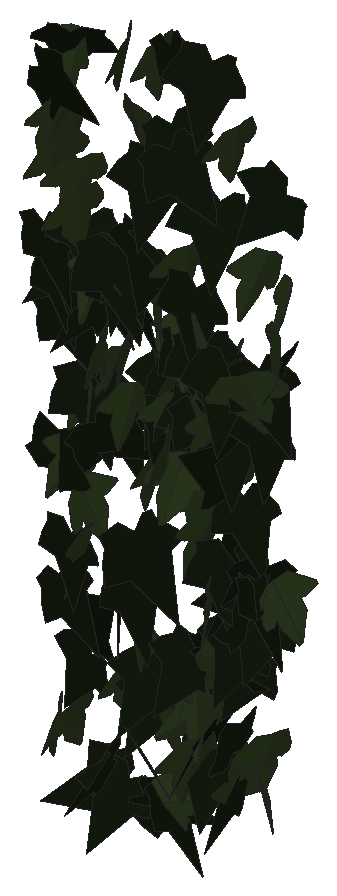
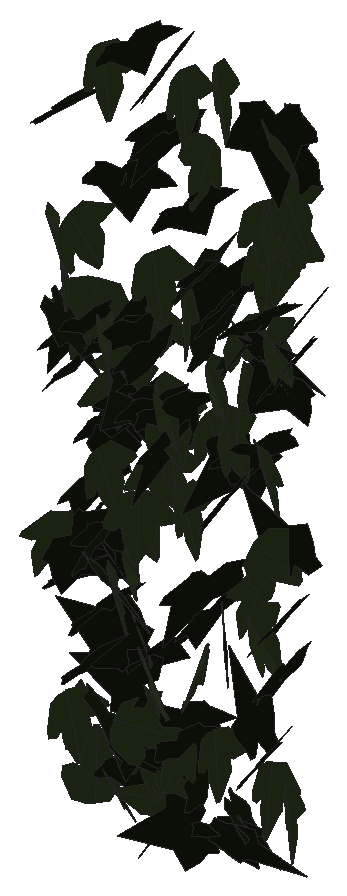
# SketchUp Ruby script. Lengths in inches.
U = 1.inch
M = Sketchup.active_model
def pt(a) = Geom::Point3d.new(a.map { |v| v * U })
def face(e, loops, mat)
  f = e.add_face(loops[0].map { |a| pt(a) })
  loops[1..].each { |l| e.add_face(l.map { |a| pt(a) }).erase! }
  f.material = f.back_material = mat if mat
  f
end
# faces: each face lists its corners as indices into pts; further lists are holes
def faces(e, pts, list, mat = nil) = list.each { |f| face(e, (f[0].is_a?(Array) ? f : [f]).map { |l| l.map { |i| pts[i] } }, mat) }
# xy, xz, yz: faces in a plane at the given z, y or x. An outline is a flat list of corners, or four numbers for a rectangle; further outlines are holes
def ring(l) = l.size == 4 ? [[l[0], l[1]], [l[2], l[1]], [l[2], l[3]], [l[0], l[3]]] : l.each_slice(2).to_a
def flat(e, list, mat, &to3) = list.each { |f| face(e, (f[0].is_a?(Array) ? f : [f]).map { |l| ring(l).map { |u, v| to3.(u, v) } }, mat) }
def xy(e, z, list, mat = nil) = flat(e, list, mat) { |x, y| [x, y, z] }
def xz(e, y, list, mat = nil) = flat(e, list, mat) { |x, z| [x, y, z] }
def yz(e, x, list, mat = nil) = flat(e, list, mat) { |y, z| [x, y, z] }
def lines(e, pts, list) = list.each { |a, b| e.add_line(pt(pts[a]), pt(pts[b])) }
# prism: a flat outline (further loops are holes) pulled along v
def prism(e, loops, v, mat = nil)
  f = face(e, loops, mat); d = Geom::Vector3d.new(v.map { |x| x * U })
  f.pushpull(f.normal.samedirection?(d) ? d.length : -d.length)
end
def box(e, o, s, mat = nil) = prism(e, [[o, [o[0] + s[0], o[1], o[2]], [o[0] + s[0], o[1] + s[1], o[2]], [o[0], o[1] + s[1], o[2]]]], [0, 0, s[2]], mat)
def at(x, y, z, deg = 0) = Geom::Transformation.translation(pt([x, y, z])) * Geom::Transformation.rotation(ORIGIN, Z_AXIS, deg.degrees)
def axes(o, x, y, z) = Geom::Transformation.new([*x, 0, *y, 0, *z, 0, *pt(o).to_a, 1])
def part(name) = M.definitions.add(name)
# library, detail: a bought-in or finely detailed component or shape, given as its bounding box
def library(name, o, s) = part(name).tap { |d| box(d.entities, o, s) }
def detail(e, o, s) = box(e.add_group.entities, o, s)
def put(e, d, t, mat = nil) = e.add_instance(d, t).tap { |i| i.material = mat if mat }
def group(e, t, mat = nil) = e.add_group.tap { |g| g.transformation = t; g.material = mat if mat }.entities
root = M.entities
M.materials.add("efeu1").color = [18, 25, 13]
M.materials.add("efeu2").color = [43, 57, 29]
c1 = part("ivyleaf_9")
p = [[1.54,2.16,1.25],[1.36,2.04,1.19],[-0.21,0.99,0.68],[-0.71,1.11,0.82],[-0.85,0.86,0.67],[-0.8,0.17,0.21],
  [-0.9,-0.01,0.1],[-0.67,-0.16,-0.02],[-0.08,-0.08,-0.05],[-0.03,-0.6,-0.4],[0.65,-0.88,-0.66],[0.83,-0.6,-0.49],
  [1.29,-0.42,-0.43],[1.8125,-0.07,-0.26],[1.21,0.44,0.15]]
faces(c1.entities,p,[[0,1,2,3,4,5,6,7,8,9,10,11,12,13,14]],"efeu1")
c2 = part("ivyleaf_10")
p = [[0,0.5,-0.03],[-0.0625,2.02,-0.43],[-0.19,2.01,-0.46],[-0.54,1.05,-0.29],[-0.52,0.625,-0.18],[-0.83,0.76,-0.28],
  [-1.16,0.64,-0.33],[-1.15,0.33,-0.24],[-0.77,-0.39,0.02],[-0.3,-0.51,0.16],[0.04,-0.48,0.23],[-0.02,2.01,-0.4375],
  [-0.06,2.01,-0.43],[0.04,-0.49,0.23],[0.67,-0.49,0.14],[1.38,0.36,-0.2],[1.375,0.51,-0.24],[0.81,0.65,-0.19],
  [0.62,0.59,-0.15],[0.6,1.09,-0.28],[0.5,1.23,-0.31]]
faces(c2.entities,p,[[0,1,2,3,4,5,6,7,8,9,10],[11,12,0,13,14,15,16,17,18,19,20]],"efeu2")
put(root,c1,axes([568.5,125.97,244.62],[-0.83297,0.49418,-0.33539],[0.23736,-0.25427,-0.96413],[-0.54805,-0.86121,0.0922]))
put(root,c1,axes([568.9,125.9,266.9],[-0.26694,-1.01056,-0.71541],[0.18661,0.69065,-1.04522],[1.22402,-0.32568,0.00333]))
put(root,c2,axes([571.5,125.46,259.34],[0.24629,-0.95429,-0.66969],[-0.13163,0.65733,-0.98509],[1.15837,0.27759,0.03045]))
put(root,c2,axes([575.38,125.65,263.47],[-0.99965,-0.67534,-0.28068],[0.21836,0.17807,-1.20614],[0.69799,-1.02292,-0.02465]))
put(root,c1,axes([576.28,126.77,271.46],[-0.55812,-0.7736,0.61929],[-0.06417,-0.68105,-0.90858],[0.98887,-0.48082,0.29057]))
put(root,c1,axes([569.01,126.375,243.78],[-0.84747,-0.6342,-0.07722],[0.05247,0.05876,-1.05838],[0.63672,-0.84895,-0.01557]))
put(root,c1,axes([569.43,126.24,252.67],[0.17619,-1.10949,-0.16604],[-0.02861,0.16358,-1.12339],[1.12148,0.17848,-0.00257]))
put(root,c1,axes([569.54,126.34,245.52],[0.51333,-0.63278,0.63099],[0.36839,-0.51313,-0.81428],[0.81416,0.63115,-0.0294]))
put(root,c2,axes([567.07,126.01,269.83],[-0.45123,-1.0268,0.03467],[-0.01509,-0.03123,-1.12157],[1.02727,-0.45148,-0.00125]))
put(root,c1,axes([565.18,126.07,273.36],[0.31586,-0.07332,-1.13873],[1.08399,0.38837,0.27567],[0.35645,-1.11608,0.17074]))
put(root,c1,axes([571.91,126.77,250.03],[-0.42919,-0.85852,0.41648],[-0.11095,-0.40867,-0.95676],[0.94774,-0.43663,0.0766]))
put(root,c2,axes([574.54,126.04,273.8],[-0.14331,-1.12142,-0.0833],[0.00662,0.08313,-1.13053],[1.12449,-0.14341,-0.00396]))
put(root,c1,axes([573.61,126.63,263.11],[-0.11921,-1.19443,0.09383],[0.00117,-0.09441,-1.20032],[1.19811,-0.11875,0.0105]))
put(root,c2,axes([572.97,126.58,253.5],[0.44592,-0.5792,0.75887],[0.50939,-0.56401,-0.7298],[0.80739,0.67574,0.04132]))
put(root,c1,axes([568,126.24,264.71],[-1.1112,0.34098,-0.19346],[0.186,-0.0533,-1.16233],[-0.3451,-1.12666,-0.00356]))
put(root,c1,axes([566.11,126.6,253.3],[0.14978,-1.03675,0.23126],[0.05339,-0.22591,-1.04732],[1.06088,0.15774,0.02006]))
put(root,c1,axes([565.09,126.35,266.4],[0.4788,-1.06287,-0.04257],[-0.0151,0.03989,-1.16573],[1.06362,0.47903,0.00262]))
put(root,c1,axes([571.64,125.85,272.1],[0.21215,-0.83368,-0.79645],[-0.02743,0.80594,-0.85092],[1.15265,0.17262,0.12634]))
put(root,c1,axes([569.57,126.97,266.68],[-0.0719,-1.03136,0.75937],[0.24506,-0.75759,-1.00574],[1.25709,0.0887,0.2395]))
put(root,c2,axes([565.98,125.95,245.71],[0.4118,-0.96484,-0.33883],[-0.06151,0.34124,-1.04646],[1.02076,0.4098,0.07364]))
put(root,c2,axes([569.19,126.43,260.52],[-0.14262,-1.03123,0.33808],[0.14789,-0.35627,-1.02434],[1.07511,-0.08779,0.18575]))
put(root,c2,axes([566.86,125.86,246.36],[-0.06368,-1.02531,-0.41092],[0.02741,0.41001,-1.02729],[1.10425,-0.0693,0.00181]))
put(root,c2,axes([575.78,126,246.45],[-0.61855,0.8704,-0.15565],[0.09102,-0.12627,-1.0678],[-0.87951,-0.62521,-0.00104]))
put(root,c2,axes([566.93,126.03,268.25],[-0.29076,-1.12264,-0.1951],[0.05471,0.18737,-1.15967],[1.13816,-0.2958,0.0059]))
put(root,c2,axes([573.18,126.61,260.73],[-0.02634,-0.95141,0.54361],[-0.01315,-0.54345,-0.95178],[1.09568,-0.02939,0.00164]))
put(root,c2,axes([572.33,126.31,246.35],[-0.18478,-1.22293,0.12241],[-0.00037,-0.12373,-1.23668],[1.22904,-0.1839,0.01803]))
put(root,c1,axes([566.09,126.18,263.6],[-0.37227,-0.2823,-1.06531],[0.90105,0.5695,-0.46578],[0.63458,-0.97424,0.03641]))
put(root,c2,axes([571.67,126.32,264.32],[1.07682,-0.16577,0.40576],[0.40215,-0.05449,-1.08948],[0.17436,1.14944,0.00687]))
put(root,c1,axes([568.35,125.47,259.4],[-0.01976,-0.17228,-1.13576],[-0.07157,1.13391,-0.17075],[1.14652,0.06782,-0.03023]))
put(root,c1,axes([573.56,126.92,258.39],[0.05127,0.06212,1.16836],[-0.71384,-0.92493,0.0805],[0.92701,-0.71568,-0.00263]))
put(root,c1,axes([568.57,126.45,243.52],[-0.96366,0.05238,0.56183],[-0.56177,0.01546,-0.96499],[-0.05305,-1.11537,0.01301]))
put(root,c1,axes([575.44,126.79,261.18],[0.04371,-1.08023,0.24664],[0.05799,-0.24427,-1.0801],[1.10651,0.05547,0.04686]))
put(root,c1,axes([575.24,126.51,254.01],[0.46177,-0.97188,0.05083],[0.02257,-0.04555,-1.076],[0.97295,0.46232,0.00083]))
put(root,c2,axes([568.11,125.83,262.56],[0.30323,-0.92257,-0.63701],[-0.02791,0.65348,-0.95971],[1.12077,0.26587,0.14845]))
put(root,c1,axes([568.38,126.91,265.87],[-0.03857,-1.05593,0.33534],[0.00439,-0.33568,-1.05651],[1.10789,-0.03543,0.01586]))
put(root,c1,axes([575.34,125.72,253.35],[-0.95299,0.20387,-0.65346],[-0.64661,0.0995,0.97404],[0.22465,1.15121,0.03153]))
put(root,c1,axes([570.99,126.3,243.89],[0.63917,-0.90924,-0.27198],[-0.15502,0.22348,-1.11142],[0.9363,0.6577,0.00165]))
put(root,c1,axes([568.43,126.72,252.19],[-0.30228,0.08526,-1.02674],[0.98425,-0.29236,-0.31405],[-0.30451,-1.02961,0.00416]))
put(root,c1,axes([567.13,126.57,260.45],[-0.05545,-1.12464,-0.42776],[0.1441,0.41893,-1.12009],[1.19458,-0.10274,0.11526]))
put(root,c2,axes([567.36,126.98,265.18],[-0.32791,-0.75345,0.73683],[0.28946,-0.80639,-0.69576],[1.01332,-0.01346,0.43718]))
put(root,c2,axes([570.72,126.06,265.18],[0.77568,-0.66922,-0.42703],[-0.08474,0.52383,-0.97484],[0.78933,0.71389,0.315]))
put(root,c2,axes([572.09,126.65,248.41],[0.99119,-0.35344,0.57322],[0.53372,-0.20974,-1.0522],[0.41067,1.12564,-0.01607]))
put(root,c2,axes([576.41,126.13,265.29],[0.72999,-0.68407,-0.49113],[-0.16509,0.52111,-0.97121],[0.82578,0.7089,0.24]))
put(root,c1,axes([568.71,126.9,264.65],[0.50735,-0.86425,0.57784],[0.32432,-0.47932,-1.00165],[0.98775,0.60129,0.03208]))
put(root,c2,axes([571.47,126.56,258.125],[0.69951,0.82364,-0.35405],[-0.26511,-0.23895,-1.07966],[-0.85642,0.74671,0.04503]))
put(root,c2,axes([571.23,125.97,243.91],[0.08297,0.05631,-1.11578],[1.04356,0.39557,0.09756],[0.39889,-1.0466,-0.02316]))
put(root,c1,axes([565.89,126.34,251.49],[0.51475,-0.89841,-0.5316],[-0.24876,0.47007,-1.0353],[1.01383,0.57149,0.01588]))
put(root,c1,axes([573.13,126.76,269.96],[-0.64882,-0.85152,-0.45532],[0.27241,0.36487,-1.07053],[0.92639,-0.70368,-0.00411]))
put(root,c1,axes([565.49,126.4375,256.17],[-0.35266,0.21256,1.08646],[0.88598,-0.62951,0.41075],[0.6638,0.95314,0.02899]))
put(root,c1,axes([572.6,126.69,263.69],[-0.18827,-0.9964,-0.41796],[0.14161,0.39785,-1.01223],[1.07119,-0.22772,0.06036]))
put(root,c1,axes([574,127.23,251.44],[-0.32456,-1.02406,0.36522],[-0.04251,-0.3689,-1.07216],[1.08641,-0.32037,0.06715]))
put(root,c1,axes([575.11,127.18,252.69],[-0.37223,-0.982,0.234],[0.13357,-0.29512,-1.02601],[1.00062,-0.32591,0.22401]))
put(root,c2,axes([573.37,126.11,250.72],[-0.22313,0.31031,0.98176],[-0.97774,0.25103,-0.30156],[-0.32275,-0.975,0.23482]))
put(root,c2,axes([565.4,126.79,271.47],[-0.06914,-1.0809,0.28869],[-0.01511,-0.28831,-1.08311],[1.11869,-0.0707,0.00322]))
put(root,c2,axes([572.38,126.94,255.87],[0.08517,-1.01726,0.47014],[0.09351,-0.4634,-1.01962],[1.11674,0.11638,0.04952]))
put(root,c1,axes([572.55,127.05,275.69],[-0.32887,-1.10495,-0.04858],[0.01058,0.04754,-1.15284],[1.10596,-0.32902,-0.00342]))
put(root,c1,axes([565.29,126.91,264.55],[0.33491,-1.09702,0.0499],[0.00066,-0.05197,-1.14691],[1.09816,0.33459,-0.01453]))
put(root,c1,axes([573.62,126.8125,254.91],[-0.29333,-1.01734,-0.37749],[0.11357,0.36011,-1.05875],[1.07916,-0.31442,0.00881]))
put(root,c2,axes([566.75,126.51,260.04],[0.87157,-0.60712,-0.24728],[-0.16709,0.19205,-1.06046],[0.63389,0.88538,0.06046]))
put(root,c2,axes([570.98,126.83,260.61],[-0.26958,-1.04797,0.25565],[0.02551,-0.26963,-1.07839],[1.0784,-0.2556,0.08941]))
put(root,c1,axes([571.71,127.17,265.54],[0.00641,-1.15086,0.10669],[0.01238,-0.10662,-1.15082],[1.15573,0.00752,0.01173]))
put(root,c2,axes([568.78,126.92,262.83],[0.54647,-0.97402,0.24753],[0.11315,-0.22034,-1.11681],[0.99859,0.55799,-0.00892]))
put(root,c2,axes([566.5,127.11,253.16],[0.44894,-1.04275,0.49477],[0.16114,-0.46906,-1.13477],[1.14288,0.47575,-0.03436]))
put(root,c1,axes([567.2,126.88,264.96],[0.62057,-0.92662,0.00007],[0.04418,0.02951,-1.11397],[0.92557,0.61987,0.05313]))
put(root,c1,axes([572.34,127.06,260.93],[-0.52443,-0.92448,-0.39502],[0.22616,0.32563,-1.06233],[0.97957,-0.57012,0.03378]))
put(root,c1,axes([566.28,127.53,247.76],[-0.15263,-0.82463,0.67572],[0.00387,-0.68304,-0.83268],[1.06611,-0.11558,0.09976]))
put(root,c2,axes([566.01,127.32,256.76],[-0.34003,-0.73045,0.74123],[-0.05753,-0.76541,-0.78067],[1.03907,-0.28141,0.19934]))
put(root,c1,axes([569.89,127.22,248.67],[-0.87468,-0.6183,-0.07224],[0.05973,0.04065,-1.07114],[0.61963,-0.87671,0.00128]))
put(root,c1,axes([572.57,127.18,246.92],[-0.51958,0.44648,-0.79608],[0.45085,-0.67094,-0.67055],[-0.79361,-0.67347,0.14026]))
put(root,c1,axes([570.05,126.36,243.49],[0.2526,0.11841,-0.99049],[0.55722,0.83074,0.24142],[0.8274,-0.59561,0.13981]))
put(root,c2,axes([568.57,126.78,275.32],[0.40855,-1.07903,-0.22505],[-0.04288,0.22427,-1.15314],[1.10141,0.40898,0.03858]))
put(root,c2,axes([565.6875,127.27,270.625],[0.24759,-1.04968,0.41802],[0.06061,-0.41498,-1.07796],[1.12823,0.25264,-0.03382]))
put(root,c1,axes([569.17,126.76,254.27],[0.23417,-1.05433,-0.74965],[-0.06459,0.75136,-1.0769],[1.29206,0.22864,0.08203]))
put(root,c1,axes([572.4,127.3,245.78],[-0.46648,-0.9233,-0.21395],[0.11617,0.18096,-1.03422],[0.94061,-0.48024,0.02163]))
put(root,c1,axes([569.6,127.5,270.03],[-0.34171,-1.10482,0.04804],[-0.02205,-0.04346,-1.15642],[1.10564,-0.34232,-0.00822]))
put(root,c2,axes([569.66,126.35,250.54],[0.43596,-0.6078,-0.72659],[0.09401,0.82366,-0.63259],[0.94261,0.19896,0.39914]))
put(root,c1,axes([573.7,127.18,244.95],[-0.84953,0.18638,-0.52079],[0.49922,-0.15267,-0.86899],[-0.2382,-0.98469,0.03615]))
put(root,c2,axes([572.07,127.65,247.5],[-0.16405,-0.42953,1.0688],[-0.39121,-0.99464,-0.45977],[1.08341,-0.42419,-0.00418]))
put(root,c1,axes([569.87,127.52,247.59],[-0.57893,-0.84086,0.1464],[-0.10895,-0.10265,-1.02041],[0.84652,-0.58827,-0.03121]))
put(root,c1,axes([571.5625,127.125,263.44],[0.14074,-1.08394,-0.35961],[-0.07941,0.35216,-1.09258],[1.13927,0.15845,-0.03173]))
put(root,c1,axes([566.45,127.28,265.27],[-1.10214,-0.03137,0.15529],[-0.15443,-0.03066,-1.10228],[0.03533,-1.1126,0.026]))
put(root,c2,axes([565.46,126.74,269.7],[-0.42158,-1.02733,-0.34535],[0.11931,0.32432,-1.1104],[1.07724,-0.43797,-0.01218]))
put(root,c1,axes([574.75,127.57,254.42],[-0.15305,0.31302,-1.12692],[0.26616,-1.09739,-0.34097],[-1.1389,-0.29852,0.07175]))
put(root,c1,axes([570.76,126.99,272.35],[0.30805,-1.0062,-0.49226],[0.00795,0.51248,-1.04257],[1.12013,0.27308,0.14278]))
put(root,c2,axes([573.14,127.7,262.64],[-0.0399,-0.23287,-1.08262],[0.37909,-1.02074,0.20559],[-1.04047,-0.36297,0.11642]))
put(root,c1,axes([574.9,127.08,263.17],[0.22658,-1.04979,-0.45449],[-0.0157,0.46042,-1.07132],[1.14384,0.21427,0.07532]))
put(root,c2,axes([573.26,127.14,252.88],[0.70893,-0.7746,-0.0278],[-0.01754,0.02163,-1.05004],[0.7749,0.70915,0.00166]))
put(root,c1,axes([572.3,126.89,260.94],[0.08033,-0.81349,-0.76492],[0.10777,0.76896,-0.80648],[1.11142,-0.01576,0.13349]))
put(root,c1,axes([573.23,127.48,260.01],[-0.08814,-1.09101,-0.08498],[0.01375,0.08414,-1.09454],[1.09423,-0.08894,0.00691]))
put(root,c2,axes([567.56,127.47,261.09],[0.19371,-0.98876,0.41748],[0.13755,-0.39785,-1.0061],[1.06443,0.23136,0.05404]))
put(root,c2,axes([575.96,127.25,266.85],[0.74681,-0.83631,0.03138],[0.01715,-0.02676,-1.12121],[0.83672,0.74699,-0.00503]))
put(root,c1,axes([572.875,127,250.27],[0.1504,-0.11983,1.045],[1.00837,-0.28394,-0.17769],[0.29929,1.01687,0.07353]))
put(root,c1,axes([570.42,127.74,261.4],[-0.54997,-0.97554,0.10136],[-0.04226,-0.09253,-1.11985],[0.97988,-0.55153,0.00859]))
put(root,c2,axes([570.23,126.97,246.94],[-0.94775,0.35185,-0.20836],[0.20485,-0.04667,-1.01059],[-0.3539,-0.96926,-0.02698]))
put(root,c1,axes([566.23,127.65,266.56],[-0.18324,-1.09774,-0.03723],[0.21219,0.00166,-1.09315],[1.07768,-0.18698,0.2089]))
put(root,c2,axes([574.57,127.64,267.54],[-0.193,-0.96134,0.57087],[0.09043,-0.59084,-0.96439],[1.1144,-0.11855,0.17712]))
put(root,c1,axes([566.26,127.5,249],[-0.24827,0.12478,1.19338],[0.63816,-1.01828,0.23923],[1.01611,0.67001,0.14134]))
put(root,c2,axes([569.74,127.28,257.48],[0.17014,-1.08677,0.02998],[0.00519,-0.02953,-1.10001],[1.08717,0.17022,0.00056]))
put(root,c1,axes([574.05,126.47,246.79],[-0.19686,0.78352,0.69383],[-0.3293,0.62377,-0.79783],[-0.99341,-0.36204,0.12698]))
put(root,c2,axes([576.09,126.77,254.18],[0.18711,1.04272,0.37326],[0.07465,0.36581,-1.05934],[-1.10499,0.20128,-0.00836]))
put(root,c1,axes([575.8,127.28,263.5625],[-0.78027,0.65891,-0.36536],[0.23012,-0.29242,-1.01883],[-0.71742,-0.81043,0.07056]))
put(root,c1,axes([572,127.16,249.11],[0.48881,-0.16923,0.92241],[0.86071,-0.33207,-0.51704],[0.37237,0.9897,-0.01575]))
put(root,c1,axes([570.5,127.27,275.59],[0.65622,-0.93043,-0.21111],[-0.09328,0.19243,-1.13805],[0.94951,0.66194,0.0341]))
put(root,c2,axes([570.84,127.45,248.67],[0.59686,-0.66051,-0.63385],[0.50535,-0.39322,0.8856],[-0.76332,-0.77678,0.09067]))
put(root,c2,axes([575.125,127.33,247.125],[-0.27623,-1.05716,0.09692],[-0.01257,-0.09688,-1.09258],[1.06152,-0.27625,0.01228]))
put(root,c1,axes([573.53,127.86,254.57],[0.22928,-0.85207,0.62346],[0.21826,-0.58595,-0.88108],[1.03299,0.31293,0.04779]))
put(root,c1,axes([570.64,127.04,259.79],[0.38433,-0.84348,-0.68833],[-0.27518,0.63099,-0.92687],[1.05335,0.4726,0.00901]))
put(root,c1,axes([573.85,127.42,257.19],[0.1071,-1.02724,-0.36339],[-0.00928,0.36426,-1.03246],[1.08958,0.10407,0.02693]))
put(root,c2,axes([565.52,127.48,274.08],[1.02932,-0.45344,0.24378],[0.23004,-0.08244,-1.12464],[0.46056,1.05458,0.0169]))
put(root,c2,axes([571.11,127.37,266.87],[-0.24959,-1.11575,0.00757],[-0.01735,-0.00388,-1.14322],[1.11564,-0.24968,-0.01608]))
put(root,c2,axes([568.96,127.125,272.28],[-1.05503,0.43932,-0.03649],[0.02974,-0.02351,-1.1428],[-0.43983,-1.0554,0.01027]))
put(root,c2,axes([570.64,127.53,261.75],[0.35067,-1.03691,0.10548],[0.02078,-0.10431,-1.09452],[1.04206,0.35102,-0.01367]))
put(root,c1,axes([565.83,126.97,274.76],[0.54387,0.81806,-0.55742],[-0.45045,-0.36183,-0.97051],[-0.88149,0.68963,0.15202]))
put(root,c2,axes([566.58,126.89,255.06],[0.04645,1.0087,0.41836],[-0.07102,0.42065,-1.00632],[-1.08971,0.01558,0.08342]))
put(root,c2,axes([568.3,127.32,247.87],[-0.08252,-1.01305,-0.15562],[-0.0022,0.1563,-1.0163],[1.02493,-0.08123,-0.01471]))
put(root,c2,axes([565.23,127.83,265.96],[0.3328,-0.94895,0.48305],[0.20146,-0.44084,-1.00482],[1.04559,0.38698,0.03986]))
put(root,c2,axes([572.75,126.85,261.88],[-0.36805,-0.47773,-0.92398],[0.62963,0.67784,-0.60127],[0.82797,-0.72783,0.04651]))
put(root,c2,axes([571.91,127.39,256.59],[-0.83079,-0.65461,0.0091],[-0.01082,-0.00096,-1.05768],[0.65458,-0.83084,-0.00594]))
put(root,c1,axes([572.69,126.5,260.99],[0.18335,0.71885,0.86475],[0.08886,0.86417,-0.73721],[-1.121,0.18607,0.083]))
put(root,c1,axes([567.55,127.61,258.67],[0.46383,-0.96056,-0.20735],[-0.06543,0.19859,-1.06635],[0.98051,0.46765,0.02693]))
put(root,c2,axes([573.28,127.75,258.1],[-0.10271,-1.03555,0.19862],[-0.00022,-0.19953,-1.04046],[1.05443,-0.10091,0.01913]))
put(root,c1,axes([573.68,128.31,249.83],[-0.34153,-0.89249,0.46777],[-0.04118,-0.48113,-0.94806],[1.0068,-0.32244,0.1199]))
put(root,c1,axes([573.75,127.37,253.36],[-0.79047,0.63904,0.28154],[-0.24981,0.13833,-1.01535],[-0.6521,-0.82763,0.04768]))
put(root,c2,axes([573.6,127.85,244.52],[-0.39896,-1.01832,-0.25647],[-0.09549,-0.23804,1.09368],[-1.04577,0.41022,-0.00202]))
put(root,c2,axes([569.61,127.57,275.08],[0.04256,-1.14133,-0.10536],[0.11849,0.10925,-1.13559],[1.14004,0.03126,0.12196]))
put(root,c1,axes([570.76,127.85,261.64],[-0.18101,-1.03258,-0.32929],[0.10191,0.31616,-1.04741],[1.07901,-0.20308,0.04369]))
